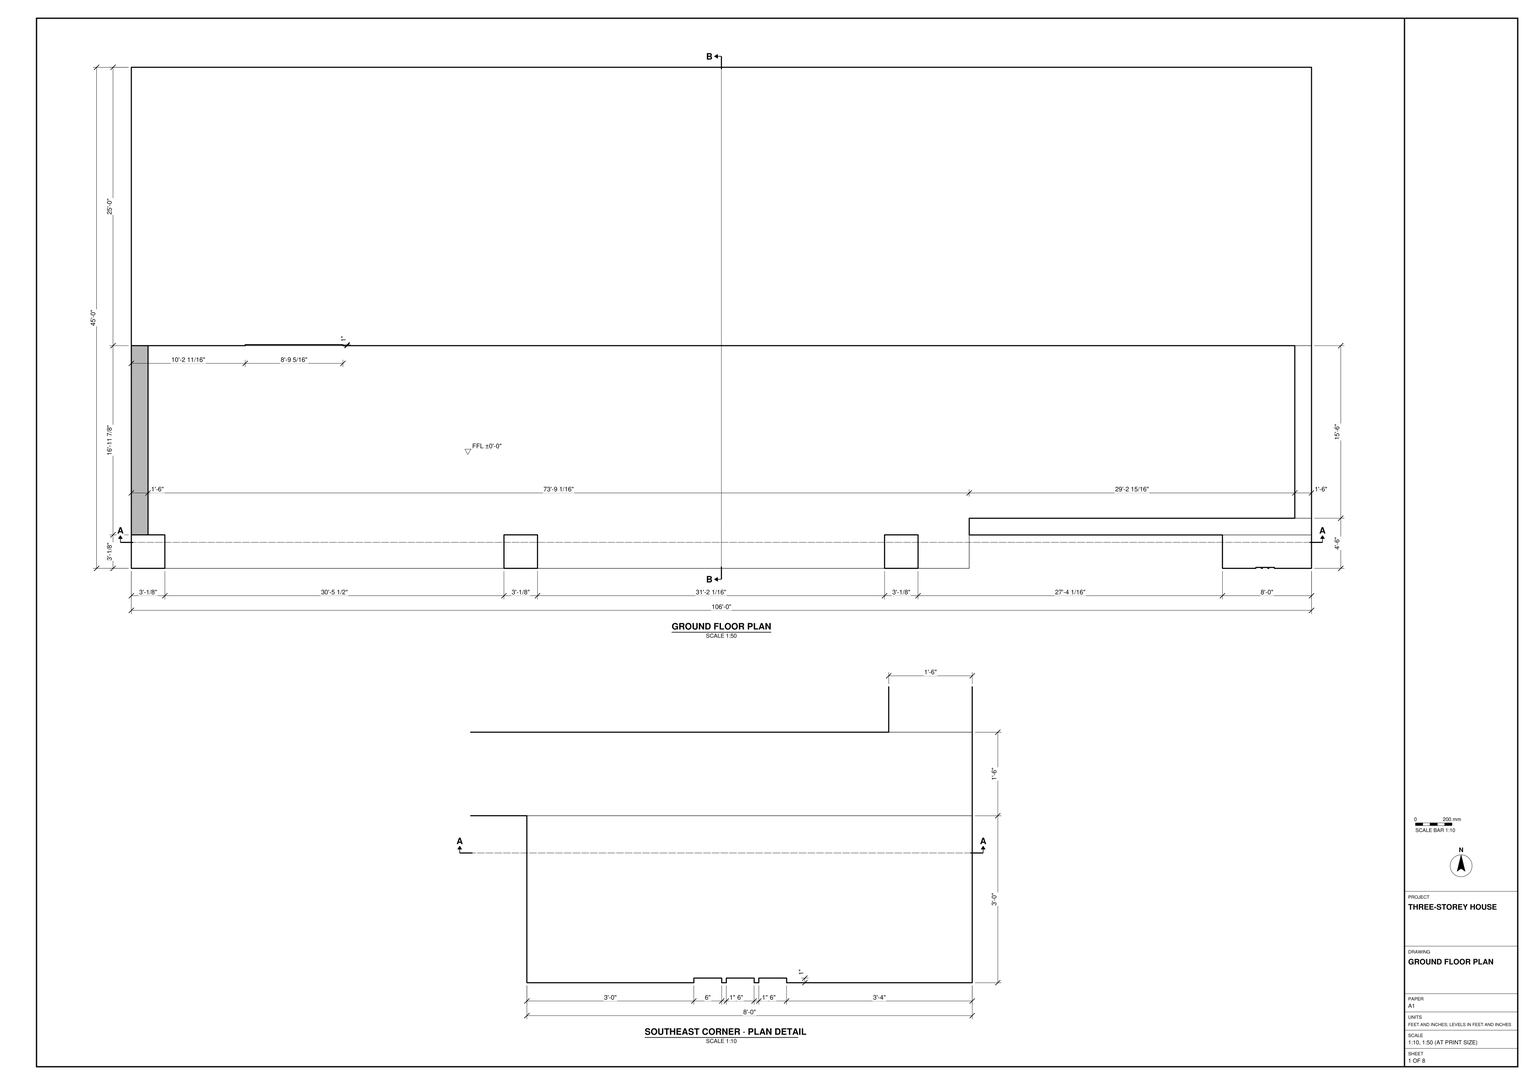
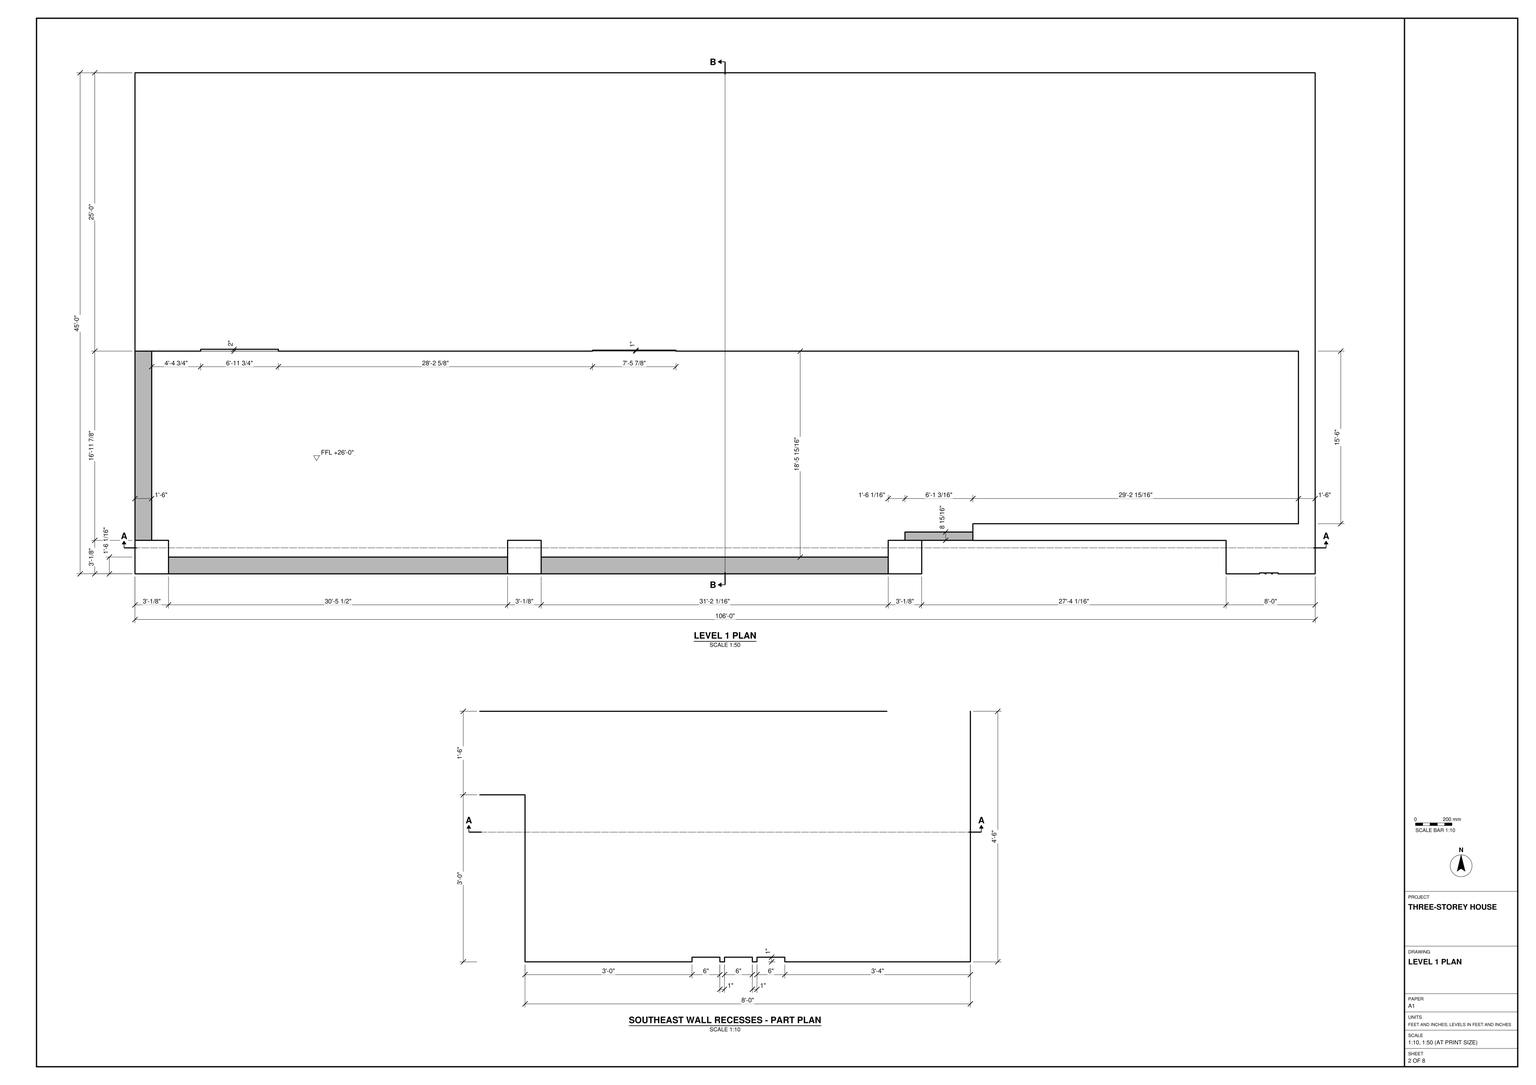
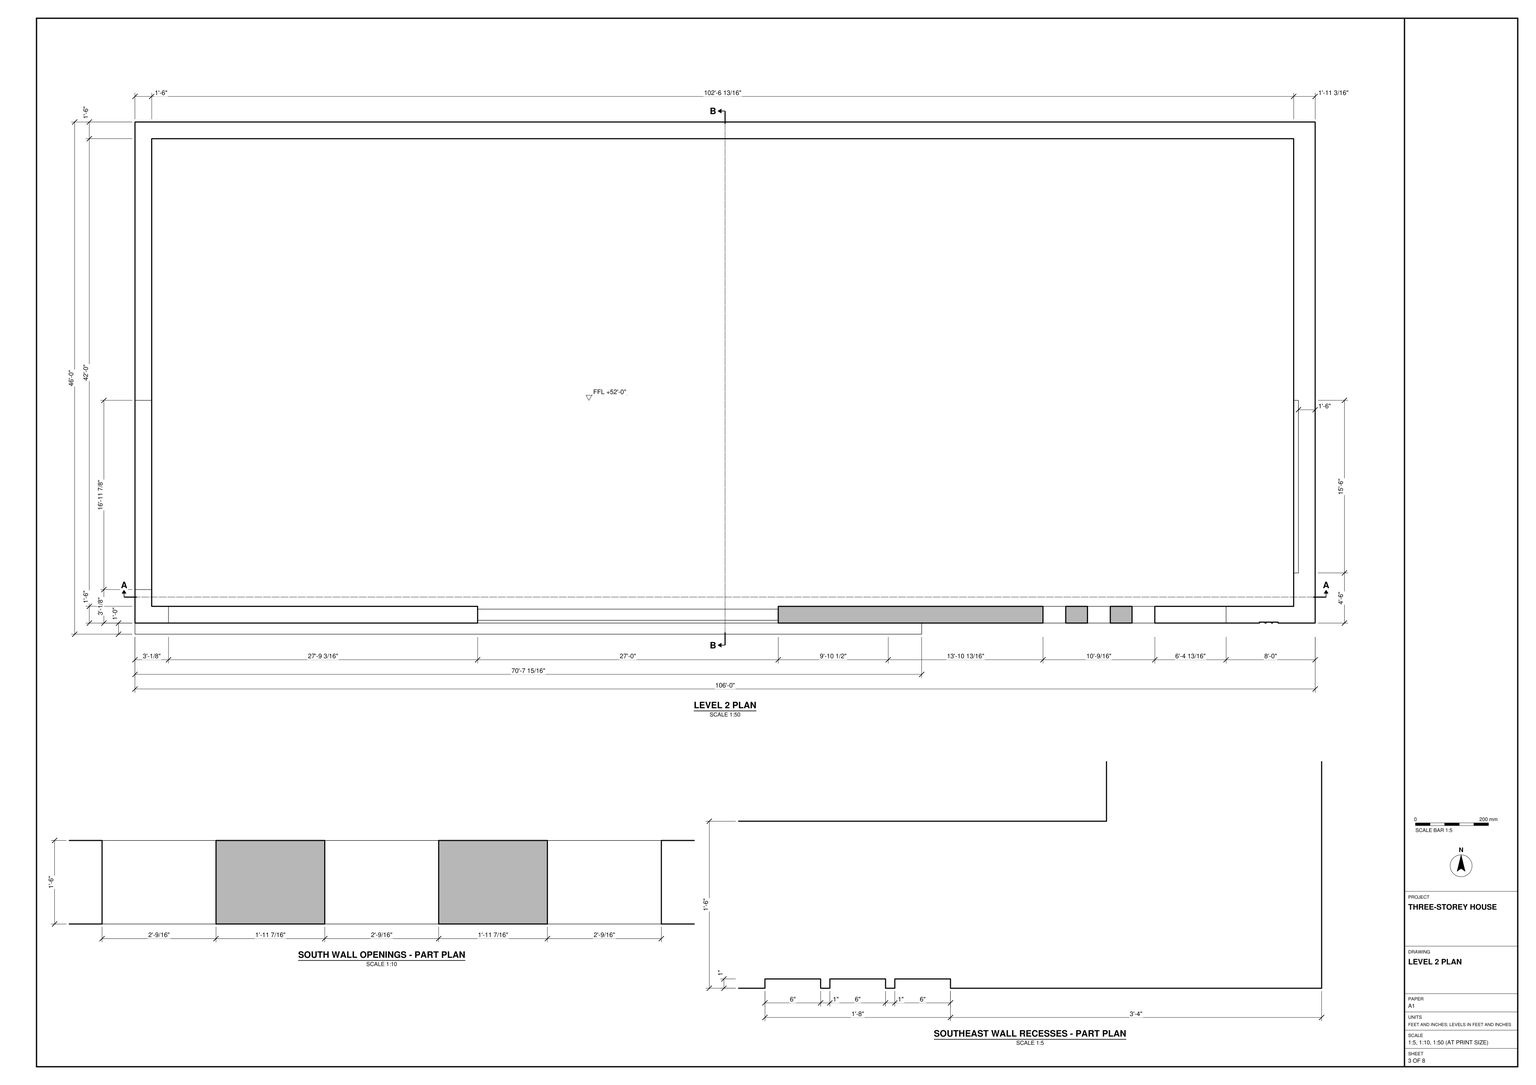
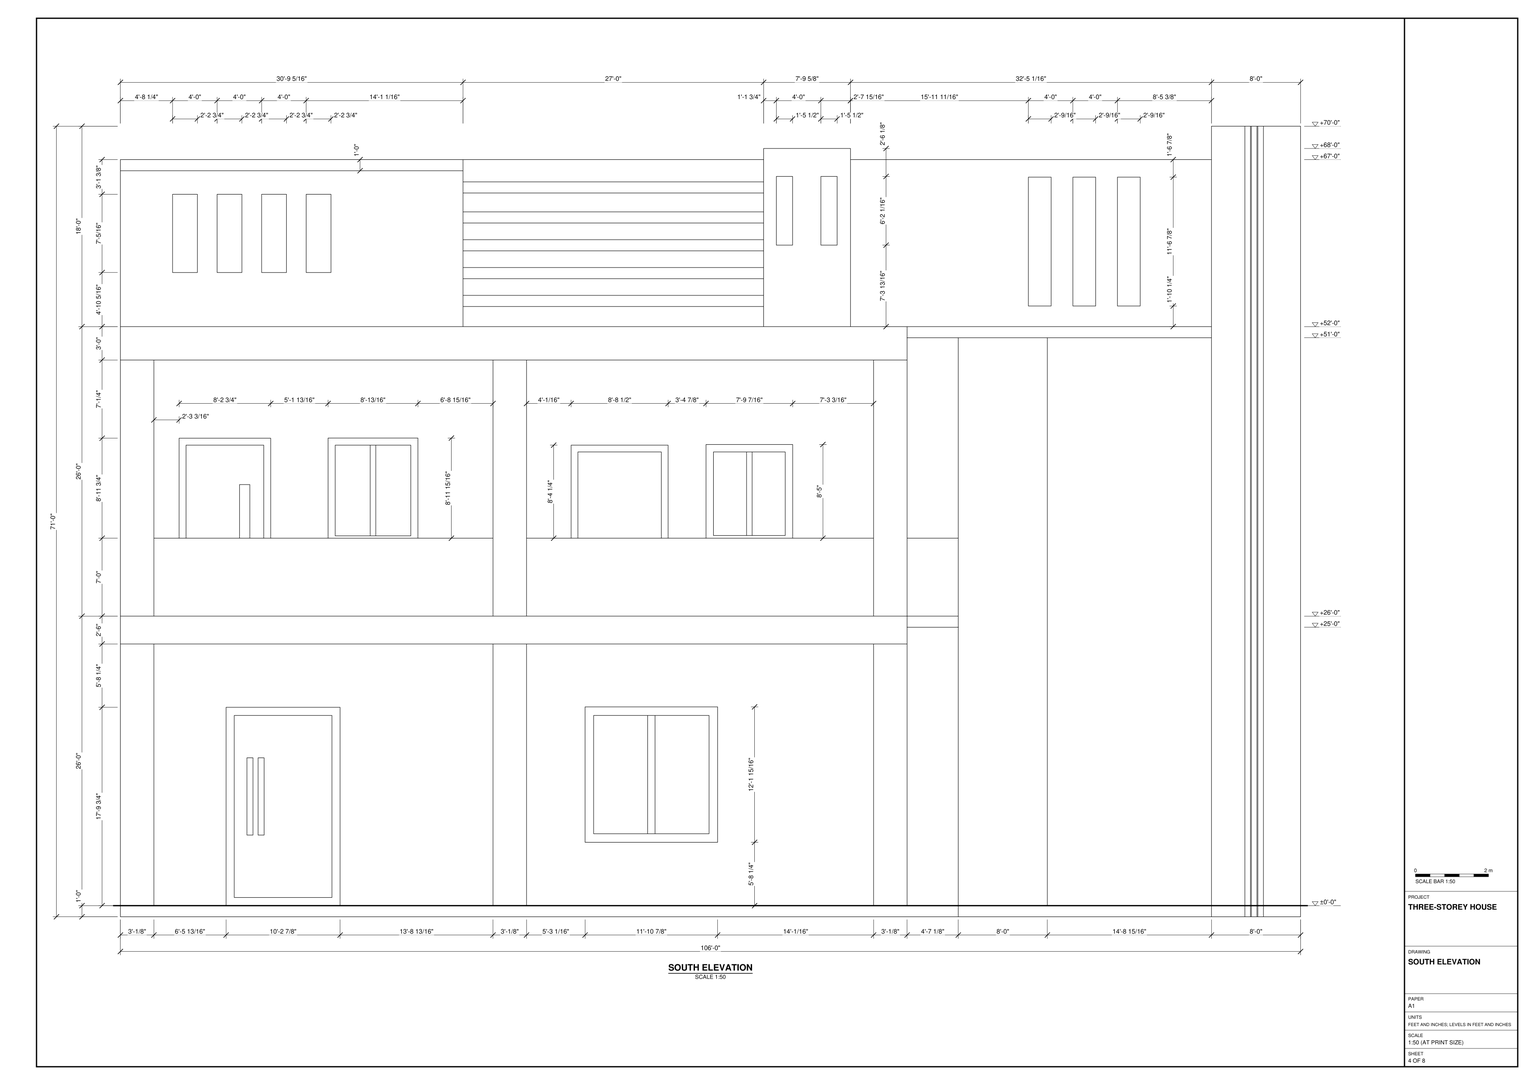
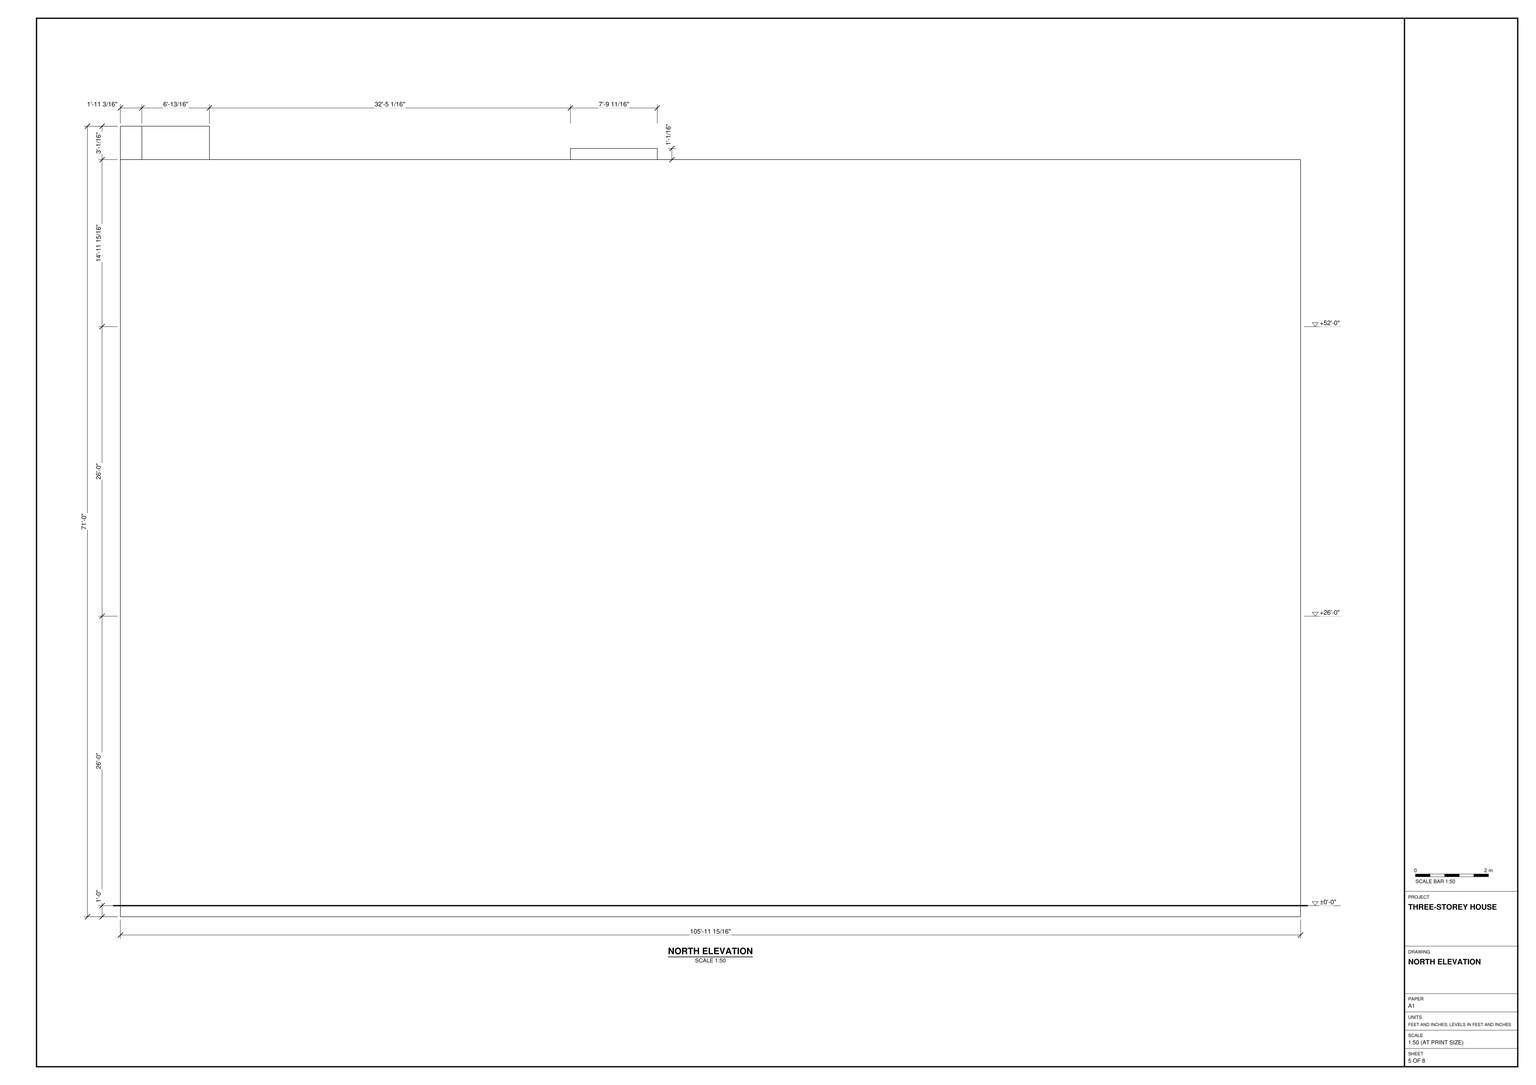
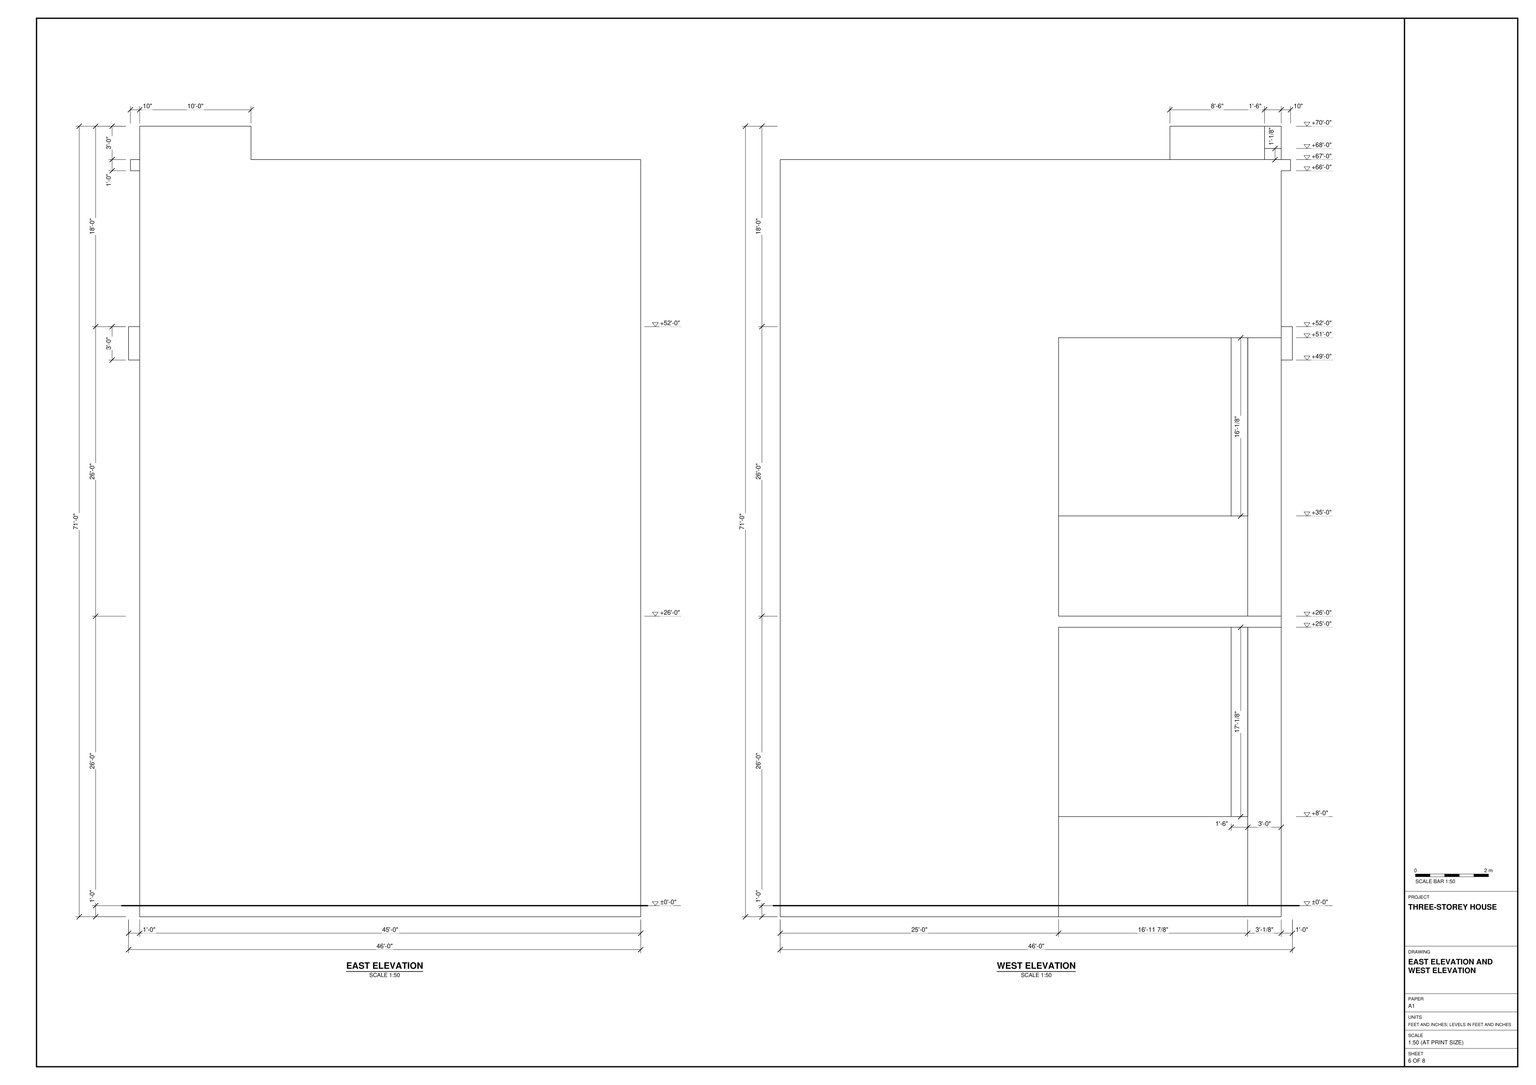
Build the three-storey house in SketchUp from task_files/diagram_01.pdf. Work in feet and inches. Set the overall extents to 106'-0" east to west, 46'-0" north to south and 71'-0" in height. Use finished floor levels of ±0'-0", +26'-0" and +52'-0" relative to the ground floor.

Use a separate plan for each storey. On the two lower storeys, set out the rear portion first, then locate the piers along the south edge and the stepped wall at the southeast corner. Include the wall sections between the piers on Level 1. Follow the enlarged plans for the shallow recesses in the southeast wall face. On Level 2, follow the perimeter wall around the floor and distinguish the broad south opening from the narrow openings farther east.

Model the walls at their drawn thicknesses and fit the floor slabs, openings and roof to the profiles shown. Include stairs, built-in joinery and main furniture only where indicated. Keep shell elements such as walls, slabs and roof, and each furniture or joinery piece, in separate groups or components; use components for repeated parts. Decor and loose items may be represented by any suitable library component. Save one SketchUp model as output_files/three_storey_house_with_a_recessed_south_frontage.skp.

# SketchUp Ruby script. Lengths in inches.
U = 1.inch
M = Sketchup.active_model
def pt(a) = Geom::Point3d.new(a.map { |v| v * U })
def face(e, loops, mat)
  f = e.add_face(loops[0].map { |a| pt(a) })
  loops[1..].each { |l| e.add_face(l.map { |a| pt(a) }).erase! }
  f.material = f.back_material = mat if mat
  f
end
# faces: each face lists its corners as indices into pts; further lists are holes
def faces(e, pts, list, mat = nil) = list.each { |f| face(e, (f[0].is_a?(Array) ? f : [f]).map { |l| l.map { |i| pts[i] } }, mat) }
# xy, xz, yz: faces in a plane at the given z, y or x. An outline is a flat list of corners, or four numbers for a rectangle; further outlines are holes
def ring(l) = l.size == 4 ? [[l[0], l[1]], [l[2], l[1]], [l[2], l[3]], [l[0], l[3]]] : l.each_slice(2).to_a
def flat(e, list, mat, &to3) = list.each { |f| face(e, (f[0].is_a?(Array) ? f : [f]).map { |l| ring(l).map { |u, v| to3.(u, v) } }, mat) }
def xy(e, z, list, mat = nil) = flat(e, list, mat) { |x, y| [x, y, z] }
def xz(e, y, list, mat = nil) = flat(e, list, mat) { |x, z| [x, y, z] }
def yz(e, x, list, mat = nil) = flat(e, list, mat) { |y, z| [x, y, z] }
def lines(e, pts, list) = list.each { |a, b| e.add_line(pt(pts[a]), pt(pts[b])) }
# prism: a flat outline (further loops are holes) pulled along v
def prism(e, loops, v, mat = nil)
  f = face(e, loops, mat); d = Geom::Vector3d.new(v.map { |x| x * U })
  f.pushpull(f.normal.samedirection?(d) ? d.length : -d.length)
end
def box(e, o, s, mat = nil) = prism(e, [[o, [o[0] + s[0], o[1], o[2]], [o[0] + s[0], o[1] + s[1], o[2]], [o[0], o[1] + s[1], o[2]]]], [0, 0, s[2]], mat)
def at(x, y, z, deg = 0) = Geom::Transformation.translation(pt([x, y, z])) * Geom::Transformation.rotation(ORIGIN, Z_AXIS, deg.degrees)
def axes(o, x, y, z) = Geom::Transformation.new([*x, 0, *y, 0, *z, 0, *pt(o).to_a, 1])
def part(name) = M.definitions.add(name)
# library, detail: a bought-in or finely detailed component or shape, given as its bounding box
def library(name, o, s) = part(name).tap { |d| box(d.entities, o, s) }
def detail(e, o, s) = box(e.add_group.entities, o, s)
def put(e, d, t, mat = nil) = e.add_instance(d, t).tap { |i| i.material = mat if mat }
def group(e, t, mat = nil) = e.add_group.tap { |g| g.transformation = t; g.material = mat if mat }.entities
root = M.entities
M.materials.add("[0012_Bisque]").color = [209, 186, 160]
M.materials.add("[0012_Bisque]1").color = [221, 198, 170]
M.materials.add("[0012_Bisque]2").color = [229, 205, 176]
M.materials.add("[0012_Bisque]3").color = [255, 228, 196]
M.materials.add("[0022_Maroon]").color = [81, 0, 0]
M.materials.add("[0111_SlateGray]").color = [79, 90, 102]
M.materials.add("[0118_Thistle]").color = [216, 191, 216]
M.materials.add("[0136_Charcoal]").color = [35, 35, 35]
M.materials.add("[Beadboard]").color = [119, 78, 49]
M.materials.add("[Granite Brown]").color = [126, 104, 91]
M.materials.add("[Stone Sandstone Ashlar Light]").color = [206, 178, 128]
M.materials.add("[Translucent Glass Gray]").color = [128, 128, 128]
M.materials["[Translucent Glass Gray]"].alpha = 0.5
M.materials.add("[Wood Cherry Original]").color = [114, 64, 31]
M.materials.add("[Wood Cherry Original]1").color = [152, 86, 42]
xy(root,0,[[0,12,0,552,1272,552,1272,66,903.08,66,903.08,12],[1176,12,1176,48,1272,48,1272,12,1232,12,1232,13,1226,13,1226,12,1225,12,1225,13,1219,13,1219,12,1218,12,1218,13,1212,13,1212,12],[903.08,48,1272,66]])
xy(root,12,[[0,12,36.125,48.125],[401.64,12,437.76,48.125],[811.8125,12,847.9375,48.125],[903.08,48,1272,66],[0,48.125,18,252],
  [1254,66,1272,252],[0,252,1272,552]])
xy(root,12,[[36.125,12,401.64,12,401.64,48.125,437.76,48.125,437.76,12,811.8125,12,811.8125,48.125,847.9375,48.125,847.9375,12,903.08,12,903.08,66,1254,66,1254,252,18,252,18,48.125,36.125,48.125]],"[Granite Brown]")
xy(root,20.78,[[122.72,252,228.03,253]])
xy(root,89.48,[[510.07,252,568.29,253],[576.29,252,634.5,253]])
xy(root,108,[[0,48.125,18,252]],"[0012_Bisque]3")
xy(root,216.97,[[122.72,252,228.03,253],[510.07,252,568.29,253],[576.29,252,634.5,253]])
xy(root,294,[[36.125,12,401.64,30.0625],[437.76,12,811.8125,30.0625]])
xy(root,312,[[847.9375,48,903.08,48.125],[152.53,79.64,149.47,80.33,146.7,81.78,144.39,83.91,142.72,86.55,141.78,89.54,141.66,92.67,142.34,95.73,143.8,98.5,145.92,100.81,148.57,102.48,151.56,103.42,154.6875,103.55,157.74,102.86,160.52,101.4,162.82,99.28,164.5,96.63,165.43,93.64,165.56,90.51,164.87,87.46,163.42,84.68,161.29,82.38,158.65,80.7,155.66,79.77],[353.84,79.64,350.78,80.33,348.01,81.78,345.7,83.91,344.03,86.55,343.1,89.54,342.97,92.67,343.65,95.73,345.11,98.5,347.23,100.81,349.88,102.48,352.87,103.42,356,103.55,359.05,102.86,361.83,101.4,364.13,99.28,365.81,96.63,366.74,93.64,366.87,90.51,366.18,87.46,364.73,84.68,362.61,82.38,359.96,80.7,356.97,79.77],[525.9,79.64,522.85,80.33,520.07,81.78,517.77,83.91,516.09,86.55,515.16,89.54,515.03,92.67,515.72,95.73,517.17,98.5,519.29,100.81,521.94,102.48,524.93,103.42,528.0625,103.55,531.12,102.86,533.89,101.4,536.2,99.28,537.87,96.63,538.8,93.64,538.93,90.51,538.25,87.46,536.79,84.68,534.67,82.38,532.02,80.7,529.03,79.77],[710.125,79.64,707.07,80.33,704.29,81.78,701.99,83.91,700.32,86.55,699.38,89.54,699.25,92.67,699.94,95.73,701.39,98.5,703.52,100.81,706.16,102.48,709.15,103.42,712.28,103.55,715.34,102.86,718.12,101.4,720.42,99.28,722.1,96.63,723.03,93.64,723.16,90.51,722.47,87.46,721.02,84.68,718.89,82.38,716.25,80.7,713.26,79.77]])
xy(root,312,[[[36.125,30.0625,36.125,48.125,0,48.125,0,252,1254,252,1254,66,903.08,66,903.08,48.125,811.8125,48.125,811.8125,30.0625,437.76,30.0625,437.76,48.125,401.64,48.125,401.64,30.0625],[353.84,79.64,356.97,79.77,359.96,80.7,362.61,82.38,364.73,84.68,366.18,87.46,366.87,90.51,366.74,93.64,365.81,96.63,364.13,99.28,361.83,101.4,359.05,102.86,356,103.55,352.87,103.42,349.88,102.48,347.23,100.81,345.11,98.5,343.65,95.73,342.97,92.67,343.1,89.54,344.03,86.55,345.7,83.91,348.01,81.78,350.78,80.33],[525.9,79.64,529.03,79.77,532.02,80.7,534.67,82.38,536.79,84.68,538.25,87.46,538.93,90.51,538.8,93.64,537.87,96.63,536.2,99.28,533.89,101.4,531.12,102.86,528.0625,103.55,524.93,103.42,521.94,102.48,519.29,100.81,517.17,98.5,515.72,95.73,515.03,92.67,515.16,89.54,516.09,86.55,517.77,83.91,520.07,81.78,522.85,80.33],[152.53,79.64,155.66,79.77,158.65,80.7,161.29,82.38,163.42,84.68,164.87,87.46,165.56,90.51,165.43,93.64,164.5,96.63,162.82,99.28,160.52,101.4,157.74,102.86,154.6875,103.55,151.56,103.42,148.57,102.48,145.92,100.81,143.8,98.5,142.34,95.73,141.66,92.67,141.78,89.54,142.72,86.55,144.39,83.91,146.7,81.78,149.47,80.33],[710.125,79.64,713.26,79.77,716.25,80.7,718.89,82.38,721.02,84.68,722.47,87.46,723.16,90.51,723.03,93.64,722.1,96.63,720.42,99.28,718.12,101.4,715.34,102.86,712.28,103.55,709.15,103.42,706.16,102.48,703.52,100.81,701.39,98.5,699.94,95.73,699.25,92.67,699.38,89.54,700.32,86.55,701.99,83.91,704.29,81.78,707.07,80.33]]],"[0118_Thistle]")
xy(root,324,[[0,12,36.125,48.125],[36.125,12,401.64,30.0625],[401.64,12,437.76,48.125],[437.76,12,811.8125,30.0625],[847.9375,48,903.08,48.125],
  [0,48.125,18,252],[829.875,48.125,903.08,57.0625]])
xy(root,324,[[36.125,30.0625,401.64,30.0625,401.64,48.125,437.76,48.125,437.76,30.0625,811.8125,30.0625,811.8125,48.125,829.875,48.125,829.875,57.0625,903.08,57.0625,903.08,66,1254,66,1254,252,18,252,18,48.125,36.125,48.125]],"[Granite Brown]")
xy(root,331.32,[[493.14,252,583.03,253]])
xy(root,331.49,[[70.78,252,154.55,254]])
xy(root,376.05,[[128.46,252,139.52,254]])
xy(root,408,[[829.875,48.125,903.08,57.0625]])
xy(root,408,[[36.125,12,401.64,30.0625],[437.76,12,811.8125,30.0625]],"[0136_Charcoal]")
xy(root,410.52,[[231.53,252,269.28,253],[275.28,252,313.02,253]])
xy(root,410.88,[[639.22,252,674.91,253],[680.91,252,716.6,253]])
xy(root,432,[[0,48.125,18,252]],"[0136_Charcoal]")
xy(root,465.8,[[128.46,252,139.52,254]])
xy(root,500.94,[[493.14,252,583.03,253],[639.22,252,674.91,253],[680.91,252,716.6,253]])
xy(root,508.26,[[70.78,252,154.55,254],[231.53,252,269.28,253],[275.28,252,313.02,253]])
xy(root,600,[[0,0,847.9375,12]])
xy(root,624,[[117.93,70.61,114.85,71.17,112.01,72.5,109.62,74.53,107.84,77.1,106.78,80.05,106.52,83.17,107.08,86.26,108.41,89.09,110.4375,91.48,113.01,93.27,115.96,94.32,119.08,94.58,122.16,94.03,125,92.6875,127.39,90.66,129.17,88.09,130.23,85.14,130.49,82.02,129.93,78.9375,128.6,76.1,126.57,73.71,124,71.93,121.05,70.87],[335.68,70.61,332.6,71.17,329.76,72.5,327.37,74.53,325.59,77.1,324.53,80.05,324.27,83.17,324.83,86.26,326.16,89.09,328.1875,91.48,330.76,93.27,333.71,94.32,336.83,94.58,339.91,94.03,342.75,92.6875,345.14,90.66,346.92,88.09,347.98,85.14,348.24,82.02,347.68,78.9375,346.35,76.1,344.32,73.71,341.75,71.93,338.8,70.87],[538.43,70.61,535.35,71.17,532.51,72.5,530.12,74.53,528.34,77.1,527.28,80.05,527.02,83.17,527.58,86.26,528.91,89.09,530.9375,91.48,533.51,93.27,536.46,94.32,539.58,94.58,542.66,94.03,545.5,92.6875,547.89,90.66,549.67,88.09,550.73,85.14,550.99,82.02,550.43,78.9375,549.1,76.1,547.07,73.71,544.5,71.93,541.55,70.87],[737.84,70.61,734.75,71.17,731.92,72.5,729.53,74.53,727.74,77.1,726.6875,80.05,726.43,83.17,726.98,86.26,728.32,89.09,730.34,91.48,732.92,93.27,735.87,94.32,738.99,94.58,742.07,94.03,744.91,92.6875,747.3,90.66,749.08,88.09,750.14,85.14,750.4,82.02,749.84,78.9375,748.5,76.1,746.48,73.71,743.91,71.93,740.96,70.87]])
xy(root,624,[[[36.125,12,36.125,48.125,0,48.125,0,252,1254,252,1254,66,903.08,66,903.08,48,1176,48,1176,12,847.9375,12,847.9375,48.125,811.8125,48.125,811.8125,12,437.76,12,437.76,48.125,401.64,48.125,401.64,12],[335.68,70.61,338.8,70.87,341.75,71.93,344.32,73.71,346.35,76.1,347.68,78.9375,348.24,82.02,347.98,85.14,346.92,88.09,345.14,90.66,342.75,92.6875,339.91,94.03,336.83,94.58,333.71,94.32,330.76,93.27,328.1875,91.48,326.16,89.09,324.83,86.26,324.27,83.17,324.53,80.05,325.59,77.1,327.37,74.53,329.76,72.5,332.6,71.17],[538.43,70.61,541.55,70.87,544.5,71.93,547.07,73.71,549.1,76.1,550.43,78.9375,550.99,82.02,550.73,85.14,549.67,88.09,547.89,90.66,545.5,92.6875,542.66,94.03,539.58,94.58,536.46,94.32,533.51,93.27,530.9375,91.48,528.91,89.09,527.58,86.26,527.02,83.17,527.28,80.05,528.34,77.1,530.12,74.53,532.51,72.5,535.35,71.17],[117.93,70.61,121.05,70.87,124,71.93,126.57,73.71,128.6,76.1,129.93,78.9375,130.49,82.02,130.23,85.14,129.17,88.09,127.39,90.66,125,92.6875,122.16,94.03,119.08,94.58,115.96,94.32,113.01,93.27,110.4375,91.48,108.41,89.09,107.08,86.26,106.52,83.17,106.78,80.05,107.84,77.1,109.62,74.53,112.01,72.5,114.85,71.17],[737.84,70.61,740.96,70.87,743.91,71.93,746.48,73.71,748.5,76.1,749.84,78.9375,750.4,82.02,750.14,85.14,749.08,88.09,747.3,90.66,744.91,92.6875,742.07,94.03,738.99,94.58,735.87,94.32,732.92,93.27,730.34,91.48,728.32,89.09,726.98,86.26,726.43,83.17,726.6875,80.05,727.74,77.1,729.53,74.53,731.92,72.5,734.75,71.17]]],"[0118_Thistle]")
xy(root,636,[[0,0,847.9375,12],[369.29,12,693.29,12,693.29,30,1248.8125,30,1248.8125,534,18,534,18,30,369.29,30]])
xy(root,658.22,[[978.62,12,1003.19,30],[1026.62,12,1051.19,30],[1074.62,12,1099.19,30]])
xy(root,694.3,[[56.25,12,83,30],[104.25,12,131,30],[152.25,12,179,30],[200.25,12,227,30]])
xy(root,723.81,[[707.01,12,724.51,14],[755.01,12,772.51,14]],"[0022_Maroon]")
xy(root,778.62,[[56.25,12,83,30],[104.25,12,131,30],[152.25,12,179,30],[200.25,12,227,30]])
xy(root,797.09,[[978.62,12,1003.19,30],[1026.62,12,1051.19,30],[1074.62,12,1099.19,30]])
xy(root,797.87,[[707.01,12,724.51,14],[755.01,12,772.51,14]],"[0022_Maroon]")
xy(root,804,[[0,2,369.29,12]],"[0136_Charcoal]")
xy(root,816,[[0,2,369.29,2,369.29,30,18,30,18,534,1248.8125,534,1248.8125,132,1272,132,1272,552,0,552],[786.9375,12,1176,30]])
xy(root,828,[[693.29,12,786.9375,30]])
xy(root,852,[[1176,12,1212,12,1212,13,1218,13,1218,12,1219,12,1219,13,1225,13,1225,12,1226,12,1226,13,1232,13,1232,12,1272,12,1272,132,1248.8125,132,1248.8125,30,1176,30]])
xz(root,0,[[0,600,847.9375,636]])
xz(root,2,[[0,804,369.29,816]],"[0136_Charcoal]")
xz(root,12,[[1218,0,1219,852],[1225,0,1226,852],[0,294,847.9375,324],[0,600,0,636,847.9375,636,847.9375,600,811.8125,600,811.8125,624,437.76,624,437.76,600,401.64,600,401.64,624,36.125,624,36.125,600],[36.125,600,401.64,624],
  [437.76,600,811.8125,624]])
xz(root,12,[[847.9375,624,1176,636],[[0,636,369.29,804],[56.25,694.3,83,778.62],[104.25,694.3,131,778.62],[200.25,694.3,227,778.62],[152.25,694.3,179,778.62]],[[693.29,636,786.9375,828],[755.01,723.81,772.51,797.87],[707.01,723.81,724.51,797.87]],[[786.9375,636,1176,816],[1074.62,658.22,1099.19,797.09],[1026.62,658.22,1051.19,797.09],[978.62,658.22,1003.19,797.09]]],"[0012_Bisque]")
xz(root,12,[[1176,0,1212,852],[1232,0,1272,852]],"[0012_Bisque]1")
xz(root,12,[[0,12,36.125,294],[401.64,12,437.76,294],[811.8125,12,847.9375,294],[0,324,36.125,600],[401.64,324,437.76,600],
  [811.8125,324,847.9375,600]],"[0111_SlateGray]")
xz(root,12,[[0,0,903.08,12]],"[Granite Brown]")
xz(root,12,[[36.125,324,401.64,408],[437.76,324,811.8125,408]],"[Translucent Glass Gray]")
xz(root,13,[[1212,0,1218,852],[1219,0,1225,852],[1226,0,1232,852]])
xz(root,14,[[707.01,723.81,724.51,797.87],[755.01,723.81,772.51,797.87]],"[0022_Maroon]")
xz(root,30,[[[18,636,369.29,816],[200.25,694.3,227,778.62],[104.25,694.3,131,778.62],[56.25,694.3,83,778.62],[152.25,694.3,179,778.62]],[[693.29,636,693.29,828,786.9375,828,786.9375,816,1176,816,1176,852,1248.8125,852,1248.8125,636],[978.62,658.22,1003.19,797.09],[1026.62,658.22,1051.19,797.09],[1074.62,658.22,1099.19,797.09]]])
xz(root,30.0625,[[36.125,294,401.64,312],[437.76,294,811.8125,312]])
xz(root,30.0625,[[36.125,324,401.64,408],[437.76,324,811.8125,408]],"[Translucent Glass Gray]")
xz(root,48,[[903.08,12,999.08,624],[847.9375,312,903.08,324]],"[0012_Bisque]")
xz(root,48,[[903.08,0,1176,12]],"[0012_Bisque]1")
xz(root,48,[[999.08,12,1176,624]],"[Beadboard]")
xz(root,48.125,[[0,12,18,108],[401.64,312,419.64,324],[419.64,312,437.76,324],[811.8125,312,847.9375,324],[0,324,18,432],
  [18,324,36.125,624],[401.64,324,437.76,624],[811.8125,324,811.8125,624,847.9375,624,847.9375,408,829.875,408,829.875,324],[829.875,324,847.9375,408],[0,432,18,624]])
xz(root,48.125,[[847.9375,324,903.08,408]],"[0012_Bisque]")
xz(root,48.125,[[18,12,18,108,0,108,0,312,36.125,312,36.125,12],[401.64,12,437.76,312],[811.8125,12,847.9375,312]],"[0111_SlateGray]")
xz(root,57.0625,[[829.875,324,903.08,408]])
xz(root,66,[[903.08,12,1254,312],[903.08,324,1254,624]])
xz(root,132,[[1248.8125,816,1272,852]])
xz(root,252,[[0,12,18,108],[128.46,376.05,139.52,465.8]])
xz(root,252,[[[18,12,113.9375,12,113.9375,225.75,236.8125,225.75,236.8125,12,1254,12,1254,312,0,312,0,108,18,108],[500.85,80.26,643.72,226.19]]],"[0012_Bisque]")
xz(root,252,[[0,324,18,432],[[18,324,63.29,324,63.29,515.75,162.04,515.75,162.04,324,485.82,324,485.82,508.26,590.35,508.26,590.35,324,1254,324,1254,624,18,624],[223.87,402.86,320.68,515.92],[631.2,402.86,724.625,508.97]],[0,432,18,624]],"[Stone Sandstone Ashlar Light]")
xz(root,252,[[[113.9375,12,236.8125,225.75],[122.72,20.78,228.03,216.97]],[[500.85,80.26,643.72,226.19],[510.07,89.48,634.5,216.97]],[568.29,89.48,576.29,216.97],[[63.29,324,162.04,515.75],[70.78,331.49,154.55,508.26]],[[485.82,324,590.35,508.26],[493.14,331.32,583.03,500.94]],
  [[223.87,402.86,320.68,515.92],[231.53,410.52,313.02,508.26]],[[631.2,402.86,724.625,508.97],[639.22,410.88,716.6,500.94]],[269.28,410.52,275.28,508.26],[674.91,410.88,680.91,500.94]],"[Wood Cherry Original]")
xz(root,253,[[136.42,88.03,142.92,171.34],[148.42,88.03,154.92,171.34]])
xz(root,253,[[510.07,89.48,568.29,216.97],[576.29,89.48,634.5,216.97],[231.53,410.52,269.28,508.26],[275.28,410.52,313.02,508.26],[639.22,410.88,674.91,500.94],
  [680.91,410.88,716.6,500.94]],"[Translucent Glass Gray]")
xz(root,253,[[[122.72,20.78,228.03,216.97],[136.42,88.03,142.92,171.34],[148.42,88.03,154.92,171.34]]],"[Wood Cherry Original]")
xz(root,253,[[493.14,331.32,583.03,500.94]],"[Wood Cherry Original]1")
xz(root,254,[[[70.78,331.49,154.55,508.26],[128.46,376.05,139.52,465.8]]],"[Wood Cherry Original]")
xz(root,534,[[18,636,1248.8125,816]])
xz(root,552,[[0,0,1272,12],[0,12,1272,816]])
yz(root,0,[[252,0,552,12],[252,12,252,312,12,312,12,324,252,324,252,624,12,624,12,804,2,804,2,816,552,816,552,12],[0,600,12,636]])
yz(root,0,[[12,0,252,12],[48.125,12,252,108]],"[0012_Bisque]3")
yz(root,0,[[12,12,48.125,312],[12,324,48.125,624]],"[0111_SlateGray]")
yz(root,0,[[48.125,324,252,432]],"[Translucent Glass Gray]")
yz(root,18,[[30,636,534,816]])
yz(root,18,[[48.125,12,252,108]],"[0012_Bisque]3")
yz(root,18,[[48.125,324,252,432]],"[Translucent Glass Gray]")
yz(root,36.125,[[12,324,30.0625,408]])
yz(root,36.125,[[12,12,48.125,12,48.125,312,30.0625,312,30.0625,294,12,294],[30.0625,324,48.125,324,48.125,624,12,624,12,408,30.0625,408]],"[0111_SlateGray]")
yz(root,56.25,[[12,694.3,30,778.62]])
yz(root,70.78,[[252,331.49,254,508.26]])
yz(root,83,[[12,694.3,30,778.62]])
yz(root,104.25,[[12,694.3,30,778.62]])
yz(root,122.72,[[252,20.78,253,216.97]])
yz(root,128.46,[[252,376.05,254,465.8]])
yz(root,131,[[12,694.3,30,778.62]])
yz(root,139.52,[[252,376.05,254,465.8]])
yz(root,152.25,[[12,694.3,30,778.62]])
yz(root,154.55,[[252,331.49,254,508.26]])
yz(root,179,[[12,694.3,30,778.62]])
yz(root,200.25,[[12,694.3,30,778.62]])
yz(root,227,[[12,694.3,30,778.62]])
yz(root,228.03,[[252,20.78,253,216.97]])
yz(root,231.53,[[252,410.52,253,508.26]])
yz(root,269.28,[[252,410.52,253,508.26]])
yz(root,275.28,[[252,410.52,253,508.26]])
yz(root,313.02,[[252,410.52,253,508.26]])
yz(root,369.29,[[[12,636,30,636,30,816,2,816,2,804,12,804],[21,657.68,19.45,657.88,18,658.48,16.76,659.43,15.8,660.68,15.2,662.125,15,663.68,15.2,665.23,15.8,666.68,16.76,667.92,18,668.875,19.45,669.47,21,669.68,22.55,669.47,24,668.875,25.24,667.92,26.2,666.68,26.8,665.23,27,663.68,26.8,662.125,26.2,660.68,25.24,659.43,24,658.48,22.55,657.88],[21,687.68,19.45,687.88,18,688.48,16.76,689.43,15.8,690.68,15.2,692.125,15,693.68,15.2,695.23,15.8,696.68,16.76,697.92,18,698.875,19.45,699.47,21,699.68,22.55,699.47,24,698.875,25.24,697.92,26.2,696.68,26.8,695.23,27,693.68,26.8,692.125,26.2,690.68,25.24,689.43,24,688.48,22.55,687.88],[21,717.68,19.45,717.88,18,718.48,16.76,719.43,15.8,720.68,15.2,722.125,15,723.68,15.2,725.23,15.8,726.68,16.76,727.92,18,728.875,19.45,729.47,21,729.68,22.55,729.47,24,728.875,25.24,727.92,26.2,726.68,26.8,725.23,27,723.68,26.8,722.125,26.2,720.68,25.24,719.43,24,718.48,22.55,717.88],[21,747.68,19.45,747.88,18,748.48,16.76,749.43,15.8,750.68,15.2,752.125,15,753.68,15.2,755.23,15.8,756.68,16.76,757.92,18,758.875,19.45,759.47,21,759.68,22.55,759.47,24,758.875,25.24,757.92,26.2,756.68,26.8,755.23,27,753.68,26.8,752.125,26.2,750.68,25.24,749.43,24,748.48,22.55,747.88],[21,780,19.45,780.2,18,780.8,16.76,781.76,15.8,783,15.2,784.45,15,786,15.2,787.55,15.8,789,16.76,790.24,18,791.2,19.45,791.8,21,792,22.55,791.8,24,791.2,25.24,790.24,26.2,789,26.8,787.55,27,786,26.8,784.45,26.2,783,25.24,781.76,24,780.8,22.55,780.2]],[21,657.68,19.45,657.88,18,658.48,16.76,659.43,15.8,660.68,15.2,662.125,15,663.68,15.2,665.23,15.8,666.68,16.76,667.92,18,668.875,19.45,669.47,21,669.68,22.55,669.47,24,668.875,25.24,667.92,26.2,666.68,26.8,665.23,27,663.68,26.8,662.125,26.2,660.68,25.24,659.43,24,658.48,22.55,657.88],[21,687.68,19.45,687.88,18,688.48,16.76,689.43,15.8,690.68,15.2,692.125,15,693.68,15.2,695.23,15.8,696.68,16.76,697.92,18,698.875,19.45,699.47,21,699.68,22.55,699.47,24,698.875,25.24,697.92,26.2,696.68,26.8,695.23,27,693.68,26.8,692.125,26.2,690.68,25.24,689.43,24,688.48,22.55,687.88],[21,717.68,19.45,717.88,18,718.48,16.76,719.43,15.8,720.68,15.2,722.125,15,723.68,15.2,725.23,15.8,726.68,16.76,727.92,18,728.875,19.45,729.47,21,729.68,22.55,729.47,24,728.875,25.24,727.92,26.2,726.68,26.8,725.23,27,723.68,26.8,722.125,26.2,720.68,25.24,719.43,24,718.48,22.55,717.88],[21,747.68,19.45,747.88,18,748.48,16.76,749.43,15.8,750.68,15.2,752.125,15,753.68,15.2,755.23,15.8,756.68,16.76,757.92,18,758.875,19.45,759.47,21,759.68,22.55,759.47,24,758.875,25.24,757.92,26.2,756.68,26.8,755.23,27,753.68,26.8,752.125,26.2,750.68,25.24,749.43,24,748.48,22.55,747.88],
  [21,780,19.45,780.2,18,780.8,16.76,781.76,15.8,783,15.2,784.45,15,786,15.2,787.55,15.8,789,16.76,790.24,18,791.2,19.45,791.8,21,792,22.55,791.8,24,791.2,25.24,790.24,26.2,789,26.8,787.55,27,786,26.8,784.45,26.2,783,25.24,781.76,24,780.8,22.55,780.2]])
yz(root,401.64,[[12,324,30.0625,408]])
yz(root,401.64,[[12,12,12,294,30.0625,294,30.0625,312,48.125,312,48.125,12],[30.0625,324,30.0625,408,12,408,12,624,48.125,624,48.125,324]],"[0111_SlateGray]")
yz(root,437.76,[[21.5,294,30.0625,312],[21.5,312,48.125,324],[12,324,21.5,408],[21.5,324,30.0625,408]])
yz(root,437.76,[[12,12,48.125,12,48.125,312,30.0625,312,30.0625,294,12,294],[30.0625,324,48.125,324,48.125,624,12,624,12,408,30.0625,408]],"[0111_SlateGray]")
yz(root,493.14,[[252,331.32,253,500.94]])
yz(root,510.07,[[252,89.48,253,216.97]])
yz(root,568.29,[[252,89.48,253,216.97]])
yz(root,576.29,[[252,89.48,253,216.97]])
yz(root,583.03,[[252,331.32,253,500.94]])
yz(root,634.5,[[252,89.48,253,216.97]])
yz(root,639.22,[[252,410.88,253,500.94]])
yz(root,674.91,[[252,410.88,253,500.94]])
yz(root,680.91,[[252,410.88,253,500.94]])
yz(root,693.29,[[[12,636,12,828,30,828,30,636,21,636,21,657.68,22.55,657.88,24,658.48,25.24,659.43,26.2,660.68,26.8,662.125,27,663.68,26.8,665.23,26.2,666.68,25.24,667.92,24,668.875,22.55,669.47,21,669.68,21,687.68,22.55,687.88,24,688.48,25.24,689.43,26.2,690.68,26.8,692.125,27,693.68,26.8,695.23,26.2,696.68,25.24,697.92,24,698.875,22.55,699.47,21,699.68,19.45,699.47,18,698.875,16.76,697.92,15.8,696.68,15.2,695.23,15,693.68,15.2,692.125,15.8,690.68,16.76,689.43,18,688.48,19.45,687.88,21,687.68,21,669.68,19.45,669.47,18,668.875,16.76,667.92,15.8,666.68,15.2,665.23,15,663.68,15.2,662.125,15.8,660.68,16.76,659.43,18,658.48,19.45,657.88,21,657.68,21,636],[21,780,22.55,780.2,24,780.8,25.24,781.76,26.2,783,26.8,784.45,27,786,26.8,787.55,26.2,789,25.24,790.24,24,791.2,22.55,791.8,21,792,19.45,791.8,18,791.2,16.76,790.24,15.8,789,15.2,787.55,15,786,15.2,784.45,15.8,783,16.76,781.76,18,780.8,19.45,780.2],[21,747.68,22.55,747.88,24,748.48,25.24,749.43,26.2,750.68,26.8,752.125,27,753.68,26.8,755.23,26.2,756.68,25.24,757.92,24,758.875,22.55,759.47,21,759.68,19.45,759.47,18,758.875,16.76,757.92,15.8,756.68,15.2,755.23,15,753.68,15.2,752.125,15.8,750.68,16.76,749.43,18,748.48,19.45,747.88],[21,717.68,22.55,717.88,24,718.48,25.24,719.43,26.2,720.68,26.8,722.125,27,723.68,26.8,725.23,26.2,726.68,25.24,727.92,24,728.875,22.55,729.47,21,729.68,19.45,729.47,18,728.875,16.76,727.92,15.8,726.68,15.2,725.23,15,723.68,15.2,722.125,15.8,720.68,16.76,719.43,18,718.48,19.45,717.88]]])
yz(root,707.01,[[12,723.81,14,797.87]],"[0022_Maroon]")
yz(root,716.6,[[252,410.88,253,500.94]])
yz(root,724.51,[[12,723.81,14,797.87]],"[0022_Maroon]")
yz(root,755.01,[[12,723.81,14,797.87]],"[0022_Maroon]")
yz(root,772.51,[[12,723.81,14,797.87]],"[0022_Maroon]")
yz(root,786.9375,[[12,816,30,828]])
yz(root,811.8125,[[12,324,30.0625,408]])
yz(root,811.8125,[[12,12,12,294,30.0625,294,30.0625,312,48.125,312,48.125,12],[30.0625,324,30.0625,408,12,408,12,624,48.125,624,48.125,324]],"[0111_SlateGray]")
yz(root,829.875,[[48.125,324,57.0625,408]])
yz(root,847.9375,[[48,312,48.125,324],[0,600,12,636]])
yz(root,847.9375,[[12,12,48.125,12,48.125,312,48,312,48,324,48.125,324,48.125,624,12,624]],"[0111_SlateGray]")
yz(root,903.08,[[48,0,66,12],[48,312,66,324],[48.125,324,57.0625,408]])
yz(root,903.08,[[48,12,66,312],[48,324,48,624,66,624,66,324,57.0625,324,57.0625,408,48.125,408,48.125,324]],"[0012_Bisque]2")
yz(root,903.08,[[12,0,48,12]],"[Granite Brown]")
yz(root,978.62,[[12,658.22,30,797.09]])
yz(root,1003.19,[[12,658.22,30,797.09]])
yz(root,1026.62,[[12,658.22,30,797.09]])
yz(root,1051.19,[[12,658.22,30,797.09]])
yz(root,1074.62,[[12,658.22,30,797.09]])
yz(root,1099.19,[[12,658.22,30,797.09]])
yz(root,1176,[[12,816,30,852]])
yz(root,1176,[[12,0,48,624]],"[0012_Bisque]")
yz(root,1212,[[12,0,13,852]])
yz(root,1218,[[12,0,13,852]])
yz(root,1219,[[12,0,13,852]])
yz(root,1225,[[12,0,13,852]])
yz(root,1226,[[12,0,13,852]])
yz(root,1232,[[12,0,13,852]])
yz(root,1248.8125,[[30,636,30,852,132,852,132,816,534,816,534,636]])
yz(root,1254,[[66,12,252,312],[66,324,252,624]],"[0012_Bisque]2")
yz(root,1272,[[12,0,552,12],[12,12,552,12,552,816,132,816,132,852,12,852]])
p = [[369.29,19.45,657.88],[369.29,21,657.68],[693.29,21,657.68],[693.29,19.45,657.88],[369.29,22.55,657.88],[693.29,22.55,657.88],
  [369.29,18,658.48],[693.29,18,658.48],[369.29,24,658.48],[693.29,24,658.48],[369.29,16.76,659.43],[693.29,16.76,659.43],
  [369.29,25.24,659.43],[693.29,25.24,659.43],[369.29,15.8,660.68],[693.29,15.8,660.68],[369.29,26.2,660.68],[693.29,26.2,660.68],
  [369.29,15.2,662.125],[693.29,15.2,662.125],[369.29,26.8,662.125],[693.29,26.8,662.125],[369.29,15,663.68],[693.29,15,663.68],
  [369.29,27,663.68],[693.29,27,663.68],[369.29,15.2,665.23],[693.29,15.2,665.23],[369.29,26.8,665.23],[693.29,26.8,665.23],
  [369.29,15.8,666.68],[693.29,15.8,666.68],[369.29,26.2,666.68],[693.29,26.2,666.68],[369.29,16.76,667.92],[693.29,16.76,667.92],
  [369.29,25.24,667.92],[693.29,25.24,667.92],[369.29,18,668.875],[693.29,18,668.875],[369.29,24,668.875],[693.29,24,668.875],
  [369.29,19.45,669.47],[693.29,19.45,669.47],[369.29,22.55,669.47],[693.29,22.55,669.47],[369.29,21,669.68],[693.29,21,669.68],
  [369.29,19.45,687.88],[369.29,21,687.68],[693.29,21,687.68],[693.29,19.45,687.88],[369.29,22.55,687.88],[693.29,22.55,687.88],
  [369.29,18,688.48],[693.29,18,688.48],[369.29,24,688.48],[693.29,24,688.48],[369.29,16.76,689.43],[693.29,16.76,689.43],
  [369.29,25.24,689.43],[693.29,25.24,689.43],[369.29,15.8,690.68],[693.29,15.8,690.68],[369.29,26.2,690.68],[693.29,26.2,690.68],
  [369.29,15.2,692.125],[693.29,15.2,692.125],[369.29,26.8,692.125],[693.29,26.8,692.125],[369.29,15,693.68],[693.29,15,693.68],
  [369.29,27,693.68],[693.29,27,693.68],[369.29,15.2,695.23],[693.29,15.2,695.23],[369.29,26.8,695.23],[693.29,26.8,695.23],
  [369.29,15.8,696.68],[693.29,15.8,696.68],[369.29,26.2,696.68],[693.29,26.2,696.68],[369.29,16.76,697.92],[693.29,16.76,697.92],
  [369.29,25.24,697.92],[693.29,25.24,697.92],[369.29,18,698.875],[693.29,18,698.875],[369.29,24,698.875],[693.29,24,698.875],
  [369.29,19.45,699.47],[693.29,19.45,699.47],[369.29,22.55,699.47],[693.29,22.55,699.47],[369.29,21,699.68],[693.29,21,699.68],
  [369.29,19.45,717.88],[369.29,21,717.68],[693.29,21,717.68],[693.29,19.45,717.88],[369.29,22.55,717.88],[693.29,22.55,717.88],
  [369.29,18,718.48],[693.29,18,718.48],[369.29,24,718.48],[693.29,24,718.48],[369.29,16.76,719.43],[693.29,16.76,719.43],
  [369.29,25.24,719.43],[693.29,25.24,719.43],[369.29,15.8,720.68],[693.29,15.8,720.68],[369.29,26.2,720.68],[693.29,26.2,720.68],
  [369.29,15.2,722.125],[693.29,15.2,722.125],[369.29,26.8,722.125],[693.29,26.8,722.125],[369.29,15,723.68],[693.29,15,723.68],
  [369.29,27,723.68],[693.29,27,723.68],[369.29,15.2,725.23],[693.29,15.2,725.23],[369.29,26.8,725.23],[693.29,26.8,725.23],
  [369.29,15.8,726.68],[693.29,15.8,726.68],[369.29,26.2,726.68],[693.29,26.2,726.68],[369.29,16.76,727.92],[693.29,16.76,727.92],
  [369.29,25.24,727.92],[693.29,25.24,727.92],[369.29,18,728.875],[693.29,18,728.875],[369.29,24,728.875],[693.29,24,728.875],
  [369.29,19.45,729.47],[693.29,19.45,729.47],[369.29,22.55,729.47],[693.29,22.55,729.47],[369.29,21,729.68],[693.29,21,729.68],
  [369.29,19.45,747.88],[369.29,21,747.68],[693.29,21,747.68],[693.29,19.45,747.88],[369.29,22.55,747.88],[693.29,22.55,747.88],
  [369.29,18,748.48],[693.29,18,748.48],[369.29,24,748.48],[693.29,24,748.48],[369.29,16.76,749.43],[693.29,16.76,749.43],
  [369.29,25.24,749.43],[693.29,25.24,749.43],[369.29,15.8,750.68],[693.29,15.8,750.68],[369.29,26.2,750.68],[693.29,26.2,750.68],
  [369.29,15.2,752.125],[693.29,15.2,752.125],[369.29,26.8,752.125],[693.29,26.8,752.125],[369.29,15,753.68],[693.29,15,753.68],
  [369.29,27,753.68],[693.29,27,753.68],[369.29,15.2,755.23],[693.29,15.2,755.23],[369.29,26.8,755.23],[693.29,26.8,755.23],
  [369.29,15.8,756.68],[693.29,15.8,756.68],[369.29,26.2,756.68],[693.29,26.2,756.68],[369.29,16.76,757.92],[693.29,16.76,757.92],
  [369.29,25.24,757.92],[693.29,25.24,757.92],[369.29,18,758.875],[693.29,18,758.875],[369.29,24,758.875],[693.29,24,758.875],
  [369.29,19.45,759.47],[693.29,19.45,759.47],[369.29,22.55,759.47],[693.29,22.55,759.47],[369.29,21,759.68],[693.29,21,759.68],
  [369.29,19.45,780.2],[369.29,21,780],[693.29,21,780],[693.29,19.45,780.2],[369.29,22.55,780.2],[693.29,22.55,780.2],
  [369.29,18,780.8],[693.29,18,780.8],[369.29,24,780.8],[693.29,24,780.8],[369.29,16.76,781.76],[693.29,16.76,781.76],
  [369.29,25.24,781.76],[693.29,25.24,781.76],[369.29,15.8,783],[693.29,15.8,783],[369.29,26.2,783],[693.29,26.2,783],
  [369.29,15.2,784.45],[693.29,15.2,784.45],[369.29,26.8,784.45],[693.29,26.8,784.45],[369.29,15,786],[693.29,15,786],
  [369.29,27,786],[693.29,27,786],[369.29,15.2,787.55],[693.29,15.2,787.55],[369.29,26.8,787.55],[693.29,26.8,787.55],
  [369.29,15.8,789],[693.29,15.8,789],[369.29,26.2,789],[693.29,26.2,789],[369.29,16.76,790.24],[693.29,16.76,790.24],
  [369.29,25.24,790.24],[693.29,25.24,790.24],[369.29,18,791.2],[693.29,18,791.2],[369.29,24,791.2],[693.29,24,791.2],
  [369.29,19.45,791.8],[693.29,19.45,791.8],[369.29,22.55,791.8],[693.29,22.55,791.8],[369.29,21,792],[693.29,21,792],
  [720,252,312],[641.57,252,324],[903.08,30,624],[903.08,30,636],[401.64,12,312],[401.64,30.0625,312],
  [811.8125,12,312],[811.8125,30.0625,312],[437.76,21.5,312],[437.76,12,312],[693.29,21,756],[693.29,21,786],
  [369.29,21,786],[693.29,21,753.68],[369.29,21,753.68],[693.29,21,723.68],[369.29,21,723.68],[693.29,21,693.68],
  [369.29,21,693.68],[693.29,21,663.68],[369.29,21,663.68]]
faces(root,p,[[0,1,2,3],[1,4,5,2],[6,0,3,7],[4,8,9,5],[10,6,7,11],[8,12,13,9],[14,10,11,15],[12,16,17,13],
  [18,14,15,19],[16,20,21,17],[22,18,19,23],[20,24,25,21],[26,22,23,27],[24,28,29,25],[30,26,27,31],[28,32,33,29],
  [34,30,31,35],[32,36,37,33],[38,34,35,39],[36,40,41,37],[42,38,39,43],[40,44,45,41],[46,42,43,47],[44,46,47,45],
  [48,49,50,51],[49,52,53,50],[54,48,51,55],[52,56,57,53],[58,54,55,59],[56,60,61,57],[62,58,59,63],[60,64,65,61],
  [66,62,63,67],[64,68,69,65],[70,66,67,71],[68,72,73,69],[74,70,71,75],[72,76,77,73],[78,74,75,79],[76,80,81,77],
  [82,78,79,83],[80,84,85,81],[86,82,83,87],[84,88,89,85],[90,86,87,91],[88,92,93,89],[94,90,91,95],[92,94,95,93],
  [96,97,98,99],[97,100,101,98],[102,96,99,103],[100,104,105,101],[106,102,103,107],[104,108,109,105],[110,106,107,111],[108,112,113,109],
  [114,110,111,115],[112,116,117,113],[118,114,115,119],[116,120,121,117],[122,118,119,123],[120,124,125,121],[126,122,123,127],[124,128,129,125],
  [130,126,127,131],[128,132,133,129],[134,130,131,135],[132,136,137,133],[138,134,135,139],[136,140,141,137],[142,138,139,143],[140,142,143,141],
  [144,145,146,147],[145,148,149,146],[150,144,147,151],[148,152,153,149],[154,150,151,155],[152,156,157,153],[158,154,155,159],[156,160,161,157],
  [162,158,159,163],[160,164,165,161],[166,162,163,167],[164,168,169,165],[170,166,167,171],[168,172,173,169],[174,170,171,175],[172,176,177,173],
  [178,174,175,179],[176,180,181,177],[182,178,179,183],[180,184,185,181],[186,182,183,187],[184,188,189,185],[190,186,187,191],[188,190,191,189],
  [192,193,194,195],[193,196,197,194],[198,192,195,199],[196,200,201,197],[202,198,199,203],[200,204,205,201],[206,202,203,207],[204,208,209,205],
  [210,206,207,211],[208,212,213,209],[214,210,211,215],[212,216,217,213],[218,214,215,219],[216,220,221,217],[222,218,219,223],[220,224,225,221],
  [226,222,223,227],[224,228,229,225],[230,226,227,231],[228,232,233,229],[234,230,231,235],[232,236,237,233],[238,234,235,239],[236,238,239,237]],"[0136_Charcoal]")
lines(root,p,[[240,241],[242,243],[244,245],[246,247],[248,249],[250,191],[251,252],[253,250],[254,253],[255,143],[256,255],[257,95],
  [258,257],[259,47],[260,259],[194,251],[191,194],[146,253],[143,146],[98,255],[95,98],[50,257],[2,259]])
